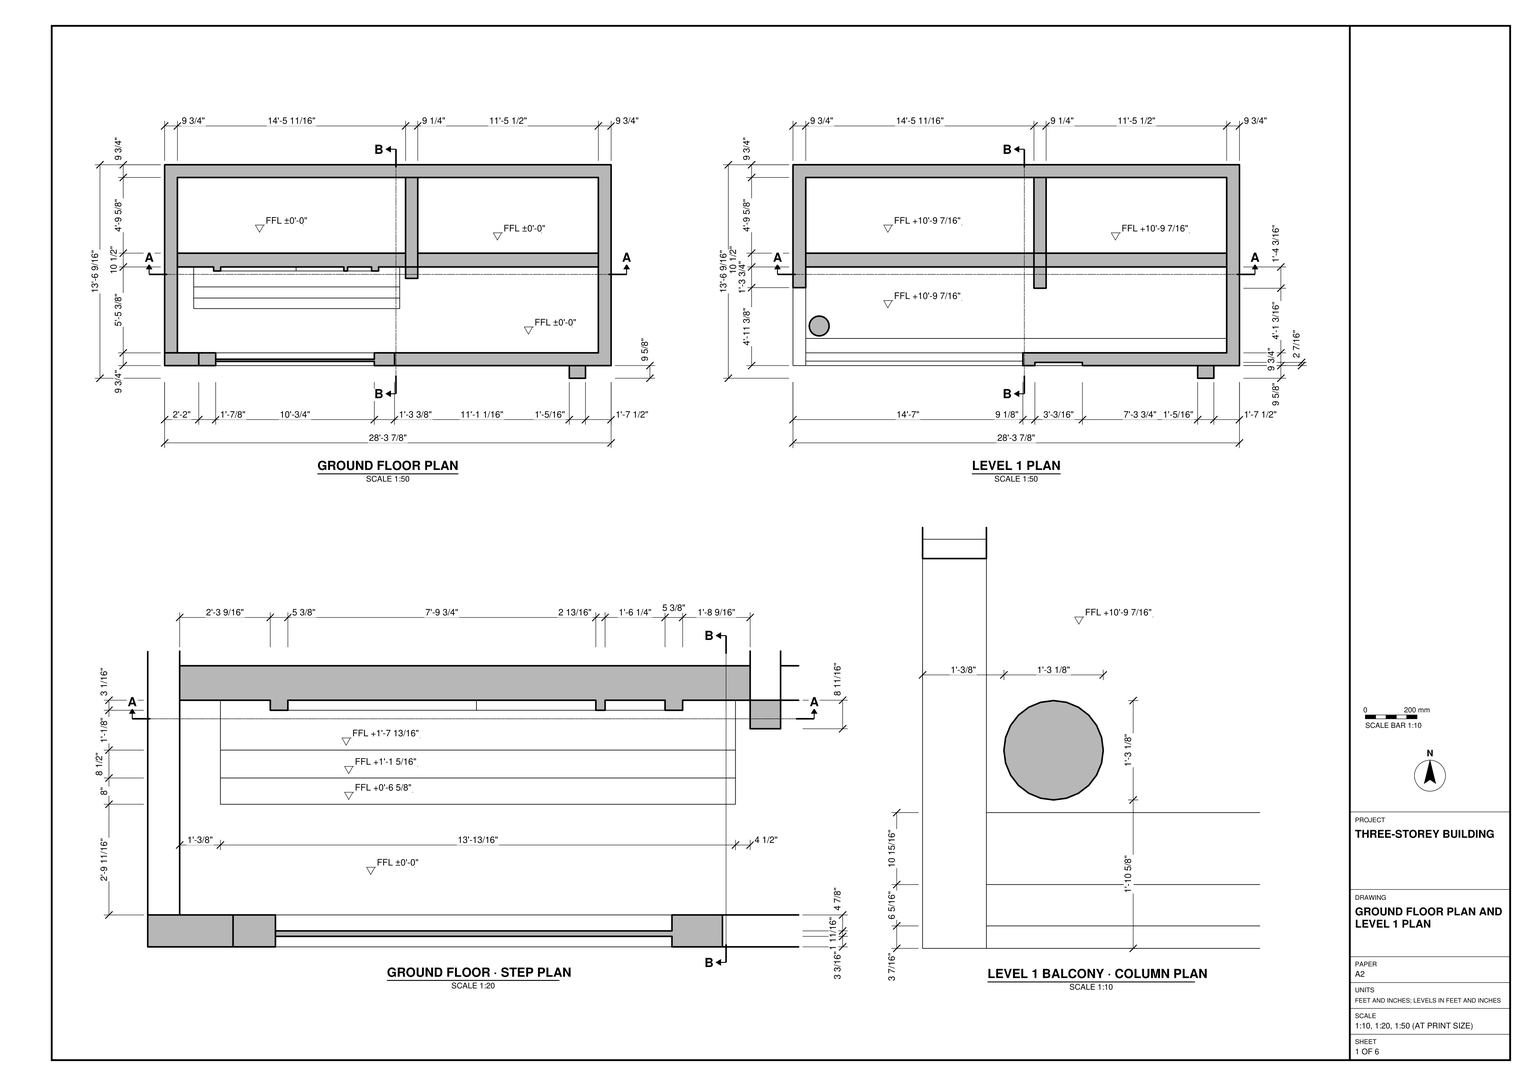
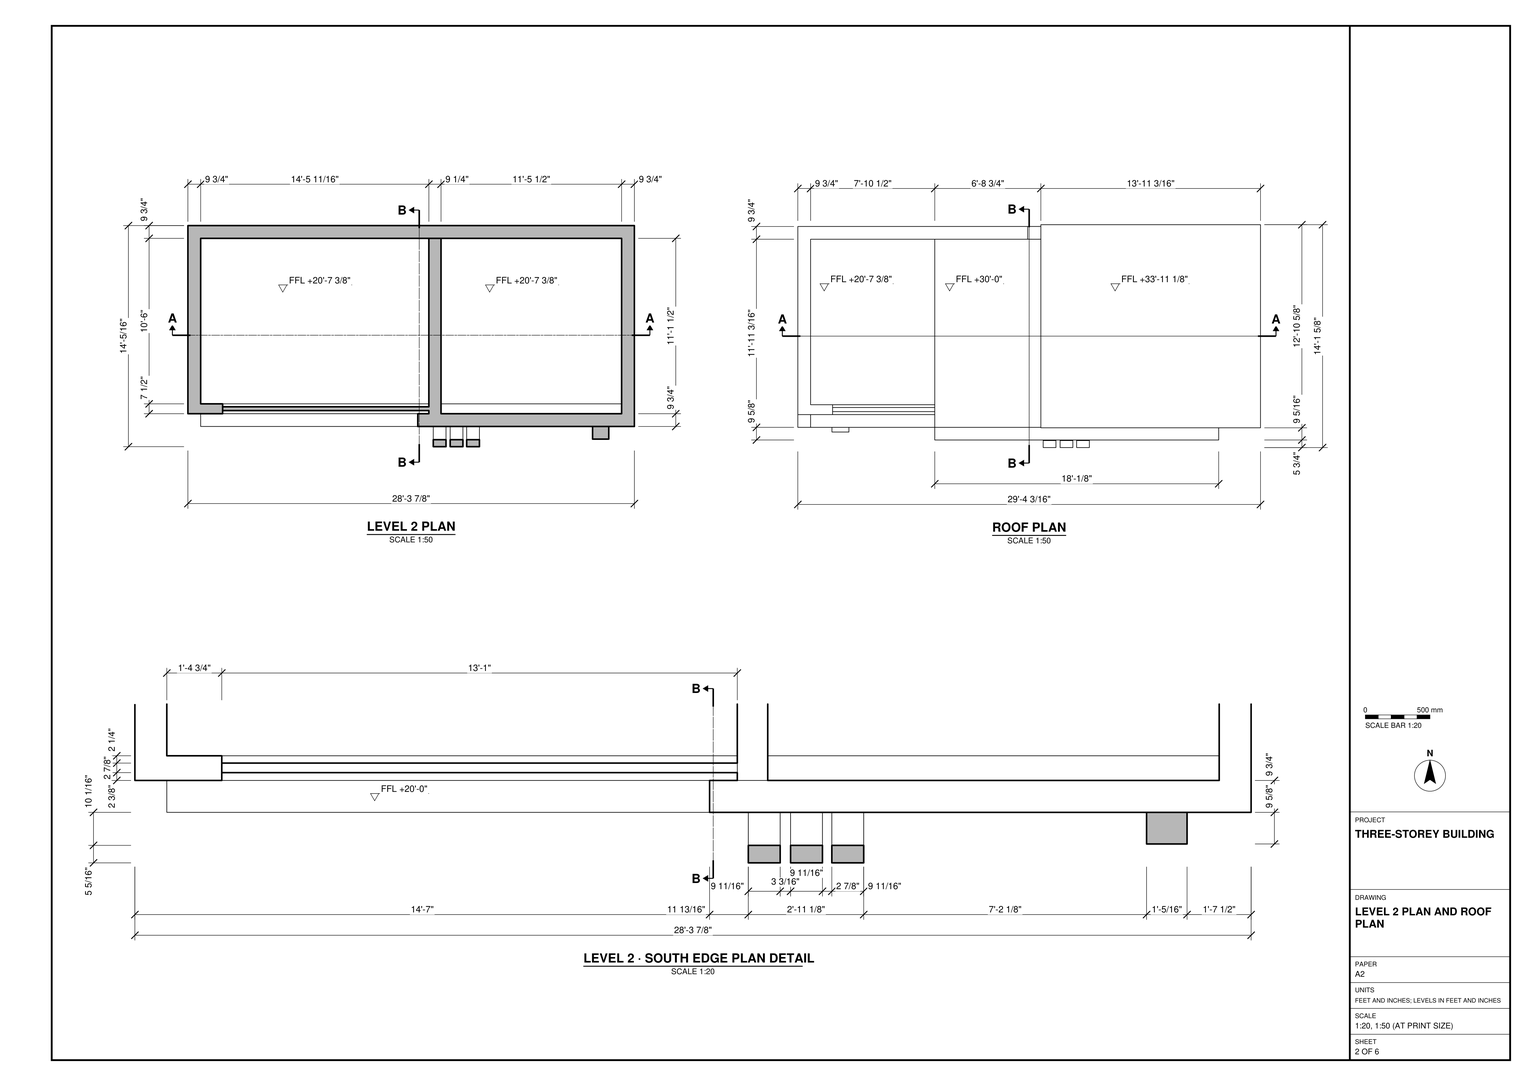
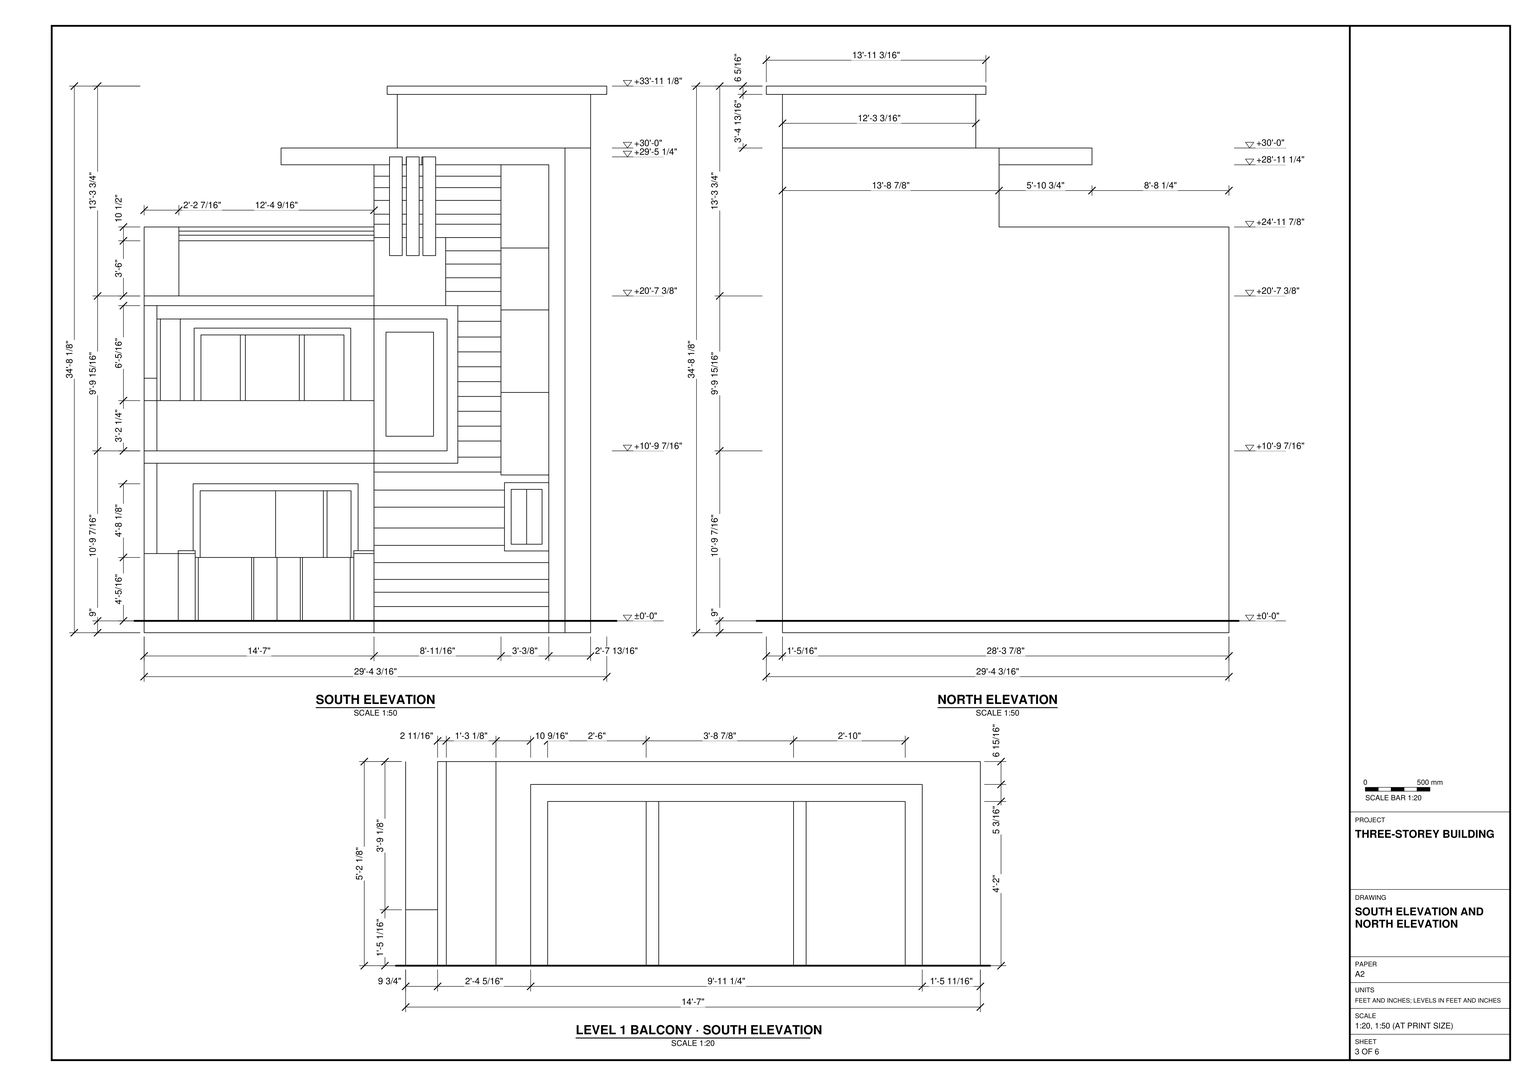
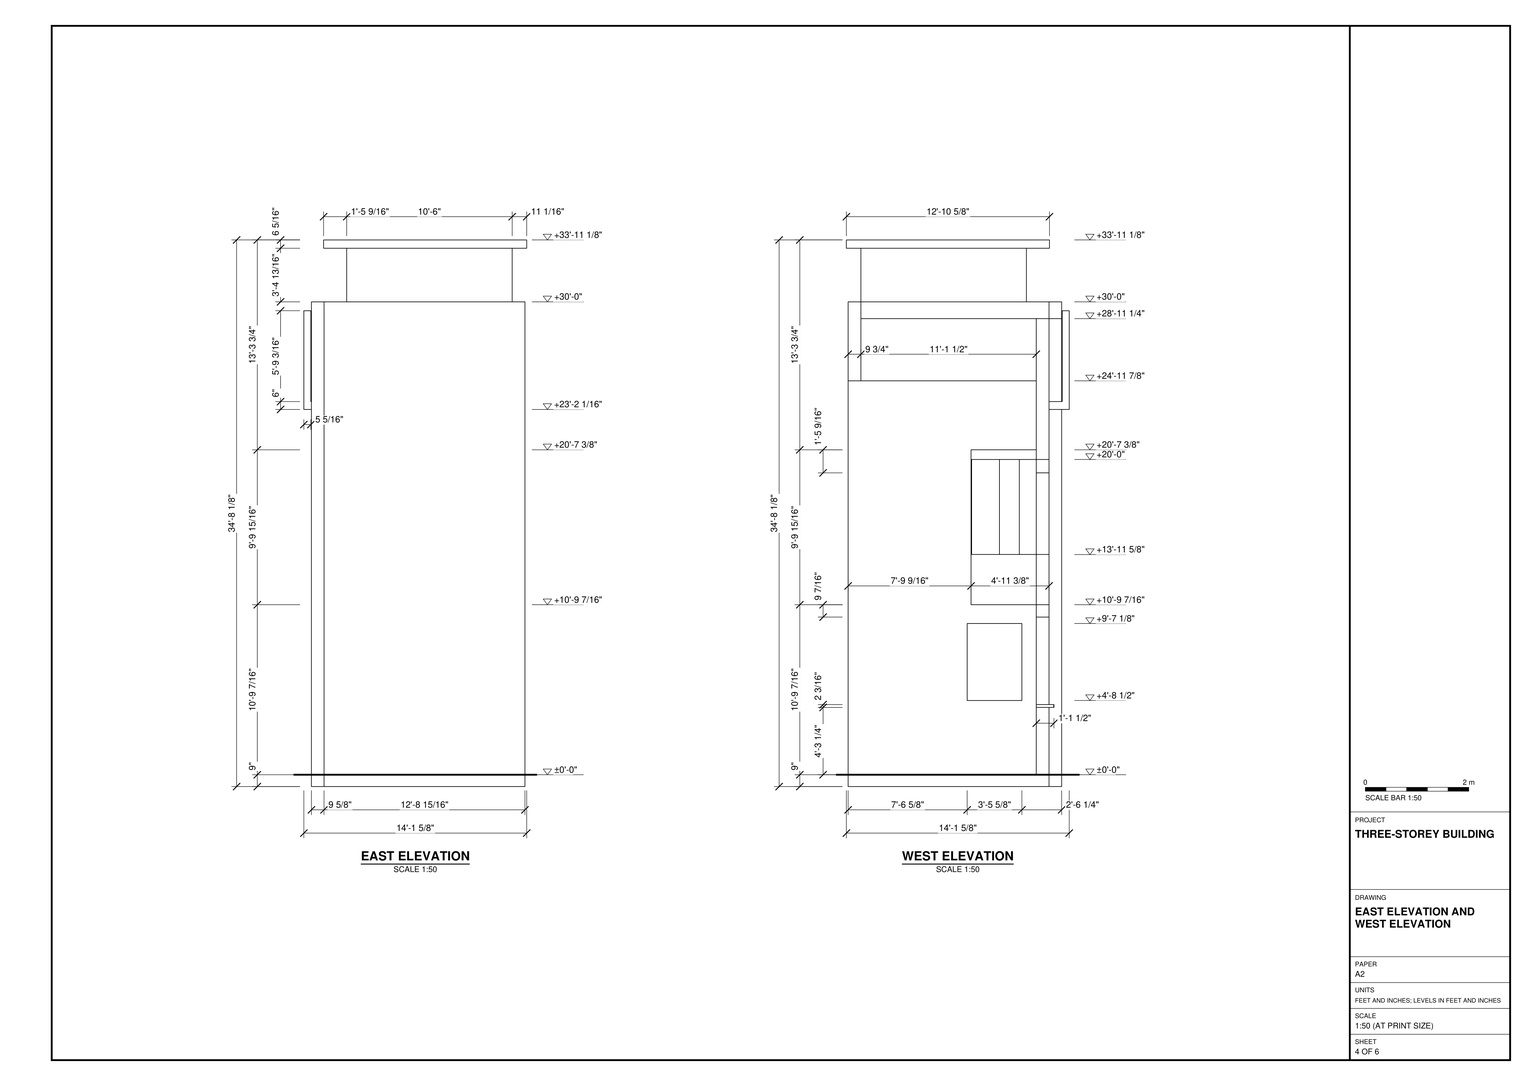
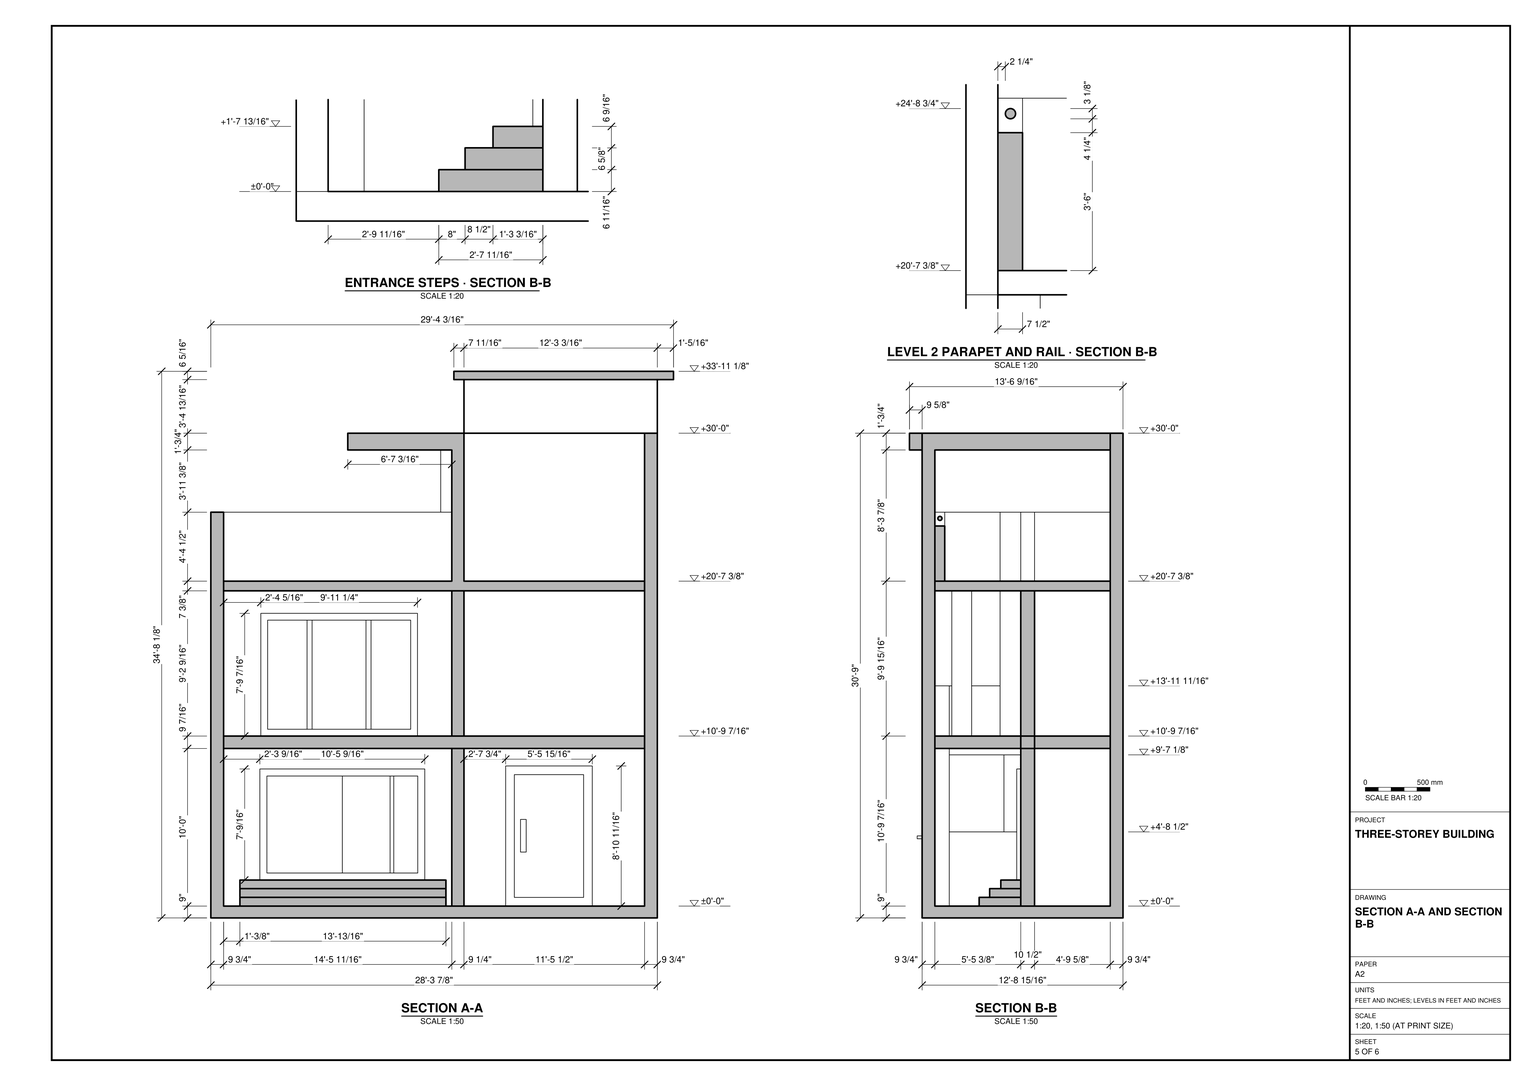
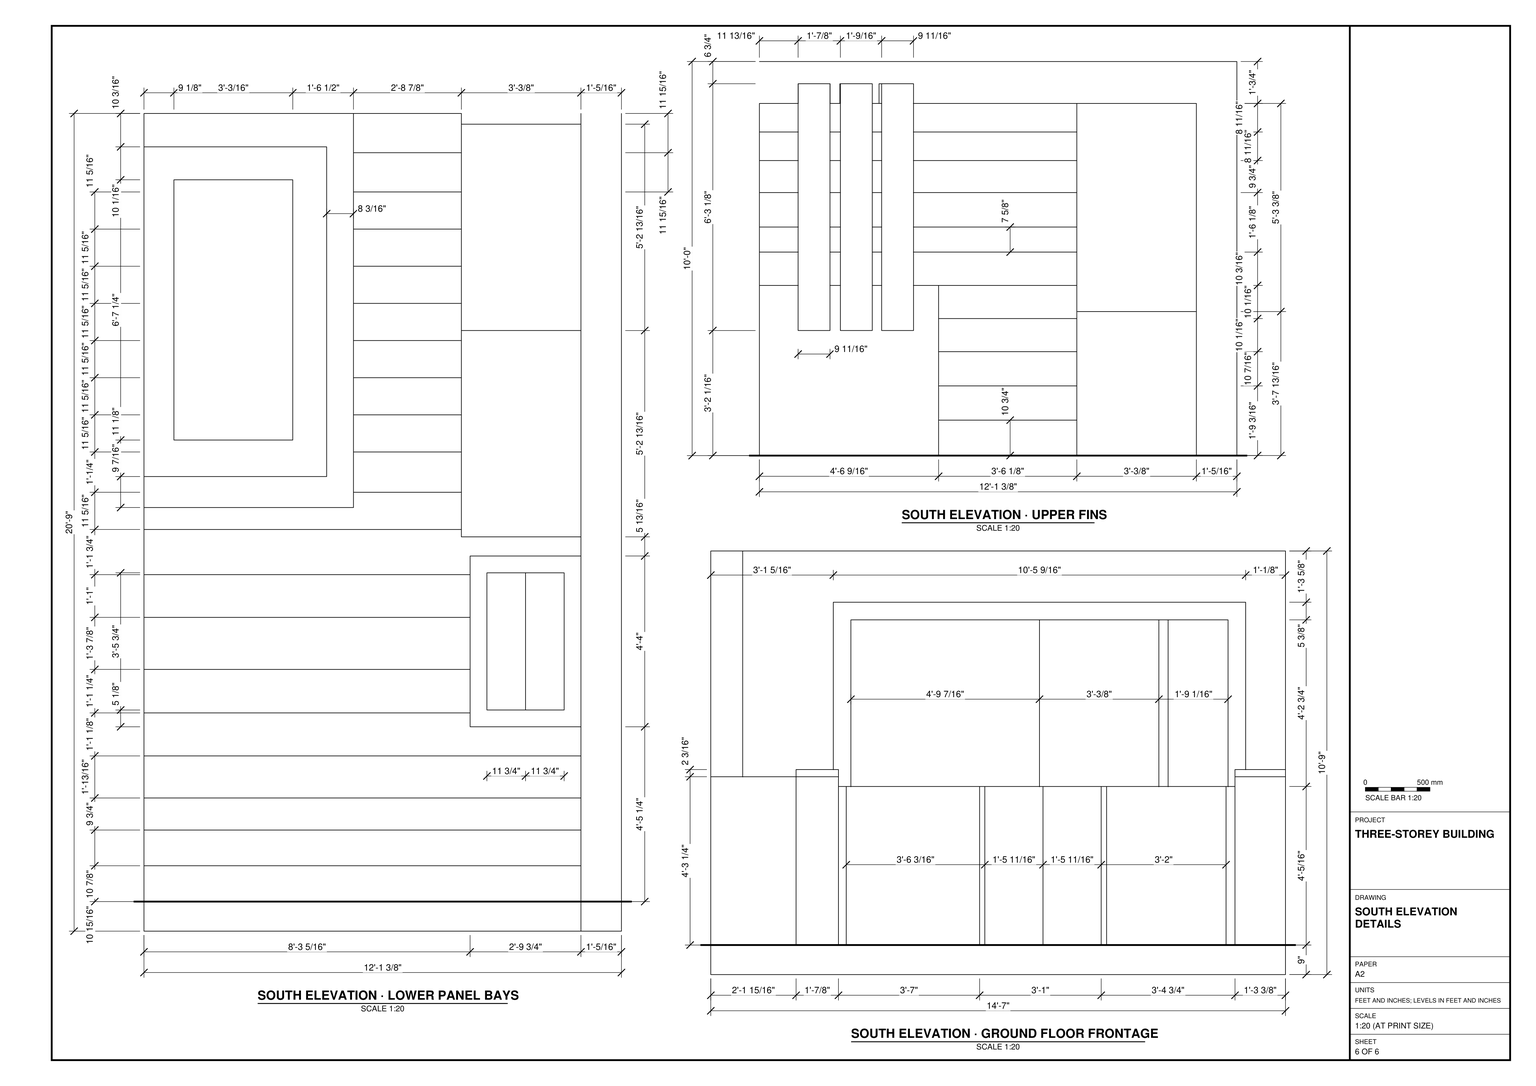
Build the three-storey building in SketchUp using task_files/diagram_01.pdf. Work in feet and inches. Set the overall dimensions to 29'-4 3/16" along the south elevation, 14'-1 5/8" from south to north and 34'-8 1/8" from the underside of the base to the top of the roof. Set the finished floor levels to ±0'-0", +10'-9 7/16" and +20'-7 3/8".

Lay out the exterior walls, internal divisions and floor slabs from the plans, keeping the wall thicknesses as drawn. In the south-west bay, model the broad ground-floor steps and the recessed balcony above them. Use the enlarged details to place the balcony column, parapet and framed opening. Follow the south elevation for the smaller ground-floor window, the projecting rectangular surround at balcony level, the horizontal bands and the three upper vertical fins. Model the open terrace and the two flat roof slabs at their distinct heights, retaining the overhangs shown in plan and elevation.

Keep walls, floor slabs and roofs in separate groups or components. Keep each furniture or joinery piece shown separate and use components for repeated parts. Any decor or loose items shown may be represented by suitable library components. Save one SketchUp model as output_files/three_storey_building_with_a_balcony_and_stepped_roof.skp.

# SketchUp Ruby script. Lengths in inches.
U = 1.inch
M = Sketchup.active_model
def pt(a) = Geom::Point3d.new(a.map { |v| v * U })
def face(e, loops, mat)
  f = e.add_face(loops[0].map { |a| pt(a) })
  loops[1..].each { |l| e.add_face(l.map { |a| pt(a) }).erase! }
  f.material = f.back_material = mat if mat
  f
end
# faces: each face lists its corners as indices into pts; further lists are holes
def faces(e, pts, list, mat = nil) = list.each { |f| face(e, (f[0].is_a?(Array) ? f : [f]).map { |l| l.map { |i| pts[i] } }, mat) }
# xy, xz, yz: faces in a plane at the given z, y or x. An outline is a flat list of corners, or four numbers for a rectangle; further outlines are holes
def ring(l) = l.size == 4 ? [[l[0], l[1]], [l[2], l[1]], [l[2], l[3]], [l[0], l[3]]] : l.each_slice(2).to_a
def flat(e, list, mat, &to3) = list.each { |f| face(e, (f[0].is_a?(Array) ? f : [f]).map { |l| ring(l).map { |u, v| to3.(u, v) } }, mat) }
def xy(e, z, list, mat = nil) = flat(e, list, mat) { |x, y| [x, y, z] }
def xz(e, y, list, mat = nil) = flat(e, list, mat) { |x, z| [x, y, z] }
def yz(e, x, list, mat = nil) = flat(e, list, mat) { |y, z| [x, y, z] }
def lines(e, pts, list) = list.each { |a, b| e.add_line(pt(pts[a]), pt(pts[b])) }
# prism: a flat outline (further loops are holes) pulled along v
def prism(e, loops, v, mat = nil)
  f = face(e, loops, mat); d = Geom::Vector3d.new(v.map { |x| x * U })
  f.pushpull(f.normal.samedirection?(d) ? d.length : -d.length)
end
def box(e, o, s, mat = nil) = prism(e, [[o, [o[0] + s[0], o[1], o[2]], [o[0] + s[0], o[1] + s[1], o[2]], [o[0], o[1] + s[1], o[2]]]], [0, 0, s[2]], mat)
def at(x, y, z, deg = 0) = Geom::Transformation.translation(pt([x, y, z])) * Geom::Transformation.rotation(ORIGIN, Z_AXIS, deg.degrees)
def axes(o, x, y, z) = Geom::Transformation.new([*x, 0, *y, 0, *z, 0, *pt(o).to_a, 1])
def part(name) = M.definitions.add(name)
# library, detail: a bought-in or finely detailed component or shape, given as its bounding box
def library(name, o, s) = part(name).tap { |d| box(d.entities, o, s) }
def detail(e, o, s) = box(e.add_group.entities, o, s)
def put(e, d, t, mat = nil) = e.add_instance(d, t).tap { |i| i.material = mat if mat }
def group(e, t, mat = nil) = e.add_group.tap { |g| g.transformation = t; g.material = mat if mat }.entities
root = M.entities
M.materials.add("[0012_Bisque]").color = [255, 228, 196]
M.materials.add("[Blinds Cellular White]").color = [217, 211, 213]
M.materials.add("[Blinds Cloth Horizontal]").color = [192, 163, 85]
M.materials.add("[Blinds Vertical Stripe Gray]").color = [160, 160, 160]
M.materials.add("[Blinds Weave]").color = [141, 91, 25]
M.materials.add("[Blinds Wood Light]").color = [155, 100, 14]
M.materials.add("[Carpet Diamond Olive]").color = [87, 77, 61]
M.materials.add("[Carpet Pattern Leaf Squares Tan]").color = [181, 154, 125]
M.materials.add("[Color M07]").color = [58, 58, 58]
M.materials.add("[Color M08]").color = [30, 30, 30]
M.materials.add("[Concrete Tile]").color = [203, 190, 164]
M.materials.add("[Formica Beige]").color = [211, 187, 149]
M.materials.add("[Formica Graystone]").color = [149, 146, 135]
M.materials.add("[Formica Laminate Dark]").color = [50, 53, 60]
M.materials.add("[Formica Laminate Light]").color = [213, 189, 164]
M.materials.add("[Formica Speckled Grey]").color = [94, 105, 111]
M.materials.add("[Metal Embossed]").color = [144, 144, 144]
M.materials.add("[Quartz Light Brown]").color = [199, 184, 152]
M.materials.add("[Stone Marble]").color = [143, 138, 136]
M.materials.add("[Translucent Glass Blue]").color = [100, 149, 237]
M.materials["[Translucent Glass Blue]"].alpha = 0.5
M.materials.add("[Translucent Glass Safety]").color = [204, 235, 244]
M.materials["[Translucent Glass Safety]"].alpha = 0.5
M.materials.add("[Wood Bamboo]").color = [177, 105, 43]
M.materials.add("[Wood Cherry Original]").color = [152, 86, 42]
M.materials.add("[Wood Floor Light]").color = [204, 176, 127]
M.materials.add("[Wood Floor Parquet]").color = [145, 89, 39]
xy(root,0,[[308.06,5.75,320.39,15.375],[0,15.375,339.89,168.31]])
xy(root,9,[[0,15.375,25.97,25.09],[25.97,15.375,38.88,25.09],[159.625,15.375,175,25.09],[38.88,18.58,159.625,20.23],[38.88,20.23,159.625,25.09],
  [22.12,58.79,178.96,90.48],[183.43,81.79,192.7,90.48],[9.72,90.48,183.43,100.97],[183.43,90.48,192.7,158.59],[192.7,90.48,330.17,100.97],
  [9.72,100.97,183.43,158.59],[192.7,100.97,330.17,158.59]])
xy(root,9,[[38.88,15.375,159.625,18.58]],"[0012_Bisque]")
xy(root,9,[[9.72,25.09,330.17,25.09,330.17,90.48,192.7,90.48,192.7,81.79,183.43,81.79,183.43,90.48,178.96,90.48,178.96,58.79,22.12,58.79,22.12,90.48,9.72,90.48]],"[Carpet Pattern Leaf Squares Tan]")
xy(root,15.65,[[22.12,66.79,178.96,90.48]])
xy(root,15.65,[[22.12,58.79,178.96,66.79]],"[Concrete Tile]")
xy(root,22.3,[[22.12,75.29,178.96,90.48]])
xy(root,22.3,[[22.12,66.79,178.96,75.29]],"[Concrete Tile]")
xy(root,28.83,[[37.31,87.42,162.87,90.48]])
xy(root,28.83,[[22.12,75.29,178.96,75.29,178.96,90.48,162.87,90.48,162.87,87.42,37.31,87.42,37.31,90.48,22.12,90.48]],"[Concrete Tile]")
xy(root,34.18,[[42.67,87.42,100.09,90.48],[100.09,87.42,136.45,90.48],[139.26,87.42,157.52,90.48]],"[Formica Laminate Dark]")
xy(root,57.28,[[38.88,18.58,159.625,20.23]],"[Color M08]")
xy(root,60.25,[[159.625,11.625,175,15.375],[25.97,11.8125,38.88,15.375],[159.625,15.375,175,25.09]])
xy(root,60.25,[[0,15.375,25.97,25.09]],"[0012_Bisque]")
xy(root,62.4375,[[159.625,11.625,175,25.09],[25.97,11.8125,38.88,25.09]],"[0012_Bisque]")
xy(root,65.5,[[0,36.05,9.72,77.67]],"[0012_Bisque]")
xy(root,108.03,[[42.67,87.42,100.09,90.48],[100.09,87.42,136.45,90.48],[139.26,87.42,157.52,90.48]],"[Formica Laminate Dark]")
xy(root,113.39,[[37.31,87.42,162.87,90.48]])
xy(root,124.14,[[0,36.05,9.72,77.67]])
xy(root,129,[[183.43,81.79,192.7,90.48],[192.7,81.79,330.17,90.48],[9.72,90.48,183.43,100.97],[183.43,90.48,192.7,100.97],[192.7,90.48,330.17,100.97],
  [9.72,100.97,183.43,158.59],[183.43,100.97,192.7,158.59],[192.7,100.97,330.17,158.59]])
xy(root,129,[[0,15.375,0,25.09,9.72,25.09,9.72,90.48,183.43,90.48,183.43,81.79,330.17,81.79,330.17,25.09,175,25.09,175,15.375]],"[Formica Laminate Light]")
xy(root,138.4375,[[0,15.375,9.72,74.73],[9.72,18.8,175,25.09],[9.72,25.09,330.17,36.05],[19.94,37.98,17.99,38.24,16.16,38.99,14.6,40.2,13.4,41.76,12.64,43.59,12.38,45.54,12.64,47.5,13.4,49.32,14.6,50.89,16.16,52.09,17.99,52.85,19.94,53.11,21.9,52.85,23.73,52.09,25.29,50.89,26.49,49.32,27.25,47.5,27.51,45.54,27.25,43.59,26.49,41.76,25.29,40.2,23.73,38.99,21.9,38.24],[183.43,74.29,192.7,90.48],
  [9.72,90.48,183.43,100.97],[183.43,90.48,192.7,100.97],[192.7,90.48,330.17,100.97],[9.72,100.97,183.43,158.59],[183.43,100.97,192.7,158.59],
  [192.7,100.97,330.17,158.59]])
xy(root,138.4375,[[9.72,15.375,175,18.8]],"[0012_Bisque]")
xy(root,138.4375,[[[9.72,36.05,330.17,36.05,330.17,90.48,192.7,90.48,192.7,74.29,183.43,74.29,183.43,90.48,9.72,90.48],[19.94,37.98,17.99,38.24,16.16,38.99,14.6,40.2,13.4,41.76,12.64,43.59,12.38,45.54,12.64,47.5,13.4,49.32,14.6,50.89,16.16,52.09,17.99,52.85,19.94,53.11,21.9,52.85,23.73,52.09,25.29,50.89,26.49,49.32,27.25,47.5,27.51,45.54,27.25,43.59,26.49,41.76,25.29,40.2,23.73,38.99,21.9,38.24]]],"[Carpet Diamond Olive]")
xy(root,149.55,[[184.12,15.375,220.3,17.8125]])
xy(root,176.6875,[[0,15.375,9.72,74.73],[9.72,18.8,175,25.09]],"[Translucent Glass Safety]")
xy(root,228.8,[[184.12,15.375,220.3,17.8125]])
xy(root,238.84,[[9.72,15.375,175,25.09]],"[Formica Laminate Light]")
xy(root,249,[[183.43,25.09,192.7,74.29],[192.7,25.09,330.17,90.48],[19.94,37.98,21.9,38.24,23.73,38.99,25.29,40.2,26.49,41.76,27.25,43.59,27.51,45.54,27.25,47.5,26.49,49.32,25.29,50.89,23.73,52.09,21.9,52.85,19.94,53.11,17.99,52.85,16.16,52.09,14.6,50.89,13.4,49.32,12.64,47.5,12.38,45.54,12.64,43.59,13.4,41.76,14.6,40.2,16.16,38.99,17.99,38.24],[183.43,74.29,192.7,90.48],[9.72,90.48,183.43,100.97],
  [183.43,90.48,192.7,100.97],[192.7,90.48,330.17,100.97],[9.72,100.97,183.43,158.59],[183.43,100.97,192.7,158.59],[192.7,100.97,330.17,158.59]])
xy(root,249,[[9.72,15.375,175,25.09]],"[0012_Bisque]")
xy(root,249,[[0,25.09,0,74.73,9.72,74.73,9.72,90.48,183.43,90.48,183.43,25.09]],"[Formica Laminate Light]")
xy(root,256.375,[[0,25.09,0,74.73,9.72,74.73,9.72,32.61,26.45,32.61,26.45,25.09],[26.45,25.09,183.43,32.61],[192.7,25.09,330.17,32.61],[9.72,32.61,183.43,158.59],[192.7,32.61,330.17,158.59]])
xy(root,287.09,[[186.78,0,196.49,15.375],[199.66,0,209.37,15.375],[212.22,0,221.93,15.375]])
xy(root,293.09,[[186.78,5.33,196.49,15.375],[199.66,5.33,209.37,15.375],[212.22,5.33,221.93,15.375]],"[Formica Speckled Grey]")
xy(root,298.375,[[26.45,25.09,183.43,32.61]],"[Translucent Glass Safety]")
xy(root,308.875,[[0,25.09,26.45,25.09,26.45,32.61,9.72,32.61,9.72,158.59,175,158.59,175,168.31,0,168.31]],"[0012_Bisque]")
xy(root,356.24,[[104.25,5.75,308.06,15.375],[104.25,15.375,175,25.09],[104.25,25.09,183.43,158.59]],"[Formica Laminate Light]")
xy(root,362.24,[[186.78,0,196.49,5.33],[199.66,0,209.37,5.33],[212.22,0,221.93,5.33]],"[Formica Speckled Grey]")
xy(root,369,[[104.25,5.75,320.39,15.375],[192.7,32.61,330.17,158.59],[330.17,32.61,339.89,158.59]])
xy(root,369,[[175,158.59,339.89,168.31]],"[Formica Beige]")
xy(root,369,[[104.25,15.375,339.89,15.375,339.89,25.09,192.7,25.09,192.7,158.59,104.25,158.59],[192.7,25.09,330.17,32.61],[330.17,25.09,339.89,32.61]],"[Formica Graystone]")
xy(root,409.8125,[[185.01,15.04,352.2,32.61],[185.01,32.61,192.7,169.65],[192.7,32.61,339.89,158.59],[339.89,32.61,352.2,169.65],[192.7,158.59,339.89,169.65]])
xy(root,416.125,[[185.01,15.04,352.2,169.65]],"[Quartz Light Brown]")
xz(root,0,[[186.78,287.09,196.49,362.24],[199.66,287.09,209.37,362.24],[212.22,287.09,221.93,362.24]],"[Formica Speckled Grey]")
xz(root,5.33,[[186.78,293.09,196.49,362.24],[199.66,293.09,209.37,362.24],[212.22,293.09,221.93,362.24]])
xz(root,5.75,[[308.06,0,320.39,0,320.39,369,104.25,369,104.25,356.24,186.82,356.24,186.82,362.24,196.52,362.24,196.52,356.24,199.5,356.24,199.5,362.24,209.21,362.24,209.21,356.24,211.43,356.24,211.43,362.24,221.13,362.24,221.13,356.24,308.06,356.24],[186.82,356.24,196.52,362.24],[199.5,356.24,209.21,362.24],[211.43,356.24,221.13,362.24]])
xz(root,11.625,[[159.625,60.25,175,62.4375]],"[0012_Bisque]")
xz(root,11.8125,[[25.97,60.25,38.88,62.4375]],"[0012_Bisque]")
xz(root,15.04,[[185.01,409.8125,352.2,416.125]],"[Quartz Light Brown]")
xz(root,15.375,[[308.06,0,308.06,356.24,104.25,356.24,104.25,369,320.39,369,320.39,0],[[274.31,62.23,308.06,114.23],[279.42,67.35,302.95,109.12]],[[175,138.4375,230.625,238.84],[184.12,149.55,220.3,228.8]],[186.78,287.09,196.49,293.09],[199.66,287.09,209.37,293.09],
  [212.22,287.09,221.93,293.09]])
xz(root,15.375,[[0,9,25.97,60.25],[25.97,9,38.88,60.25],[159.625,9,175,60.25],[0,129,175,138.4375],[175,129,238.79,129,238.79,249,175,249,175,238.84,230.625,238.84,230.625,138.4375,175,138.4375],
  [9.72,238.84,175,249]],"[0012_Bisque]")
xz(root,15.375,[[279.42,67.35,291.18,109.12],[291.18,67.35,302.95,109.12]],"[Blinds Vertical Stripe Gray]")
xz(root,15.375,[[320.39,0,339.89,369],[[175,249,229.56,300.8125],[186.78,287.09,196.49,293.09],[199.66,287.09,209.37,293.09],[212.22,287.09,221.93,293.09]]],"[Formica Graystone]")
xz(root,15.375,[[271.65,120.07,308.06,182.9],[271.65,182.9,308.06,245.73],[271.65,245.73,308.06,292.86],[271.65,292.86,308.06,356.24]],"[Translucent Glass Blue]")
xz(root,15.375,[[0,138.4375,9.72,176.6875]],"[Translucent Glass Safety]")
xz(root,15.375,[[0,0,175,9],[175,0,308.06,9],[175,9,308.06,19.92],[175,19.92,308.06,30.79],[175,30.79,308.06,40.55],
  [175,40.55,308.06,53.37],[175,53.37,308.06,53.37,308.06,62.23,274.31,62.23,274.31,66.46,175,66.46],[175,66.46,274.31,79.71],[175,79.71,274.31,95.55],[175,95.55,274.31,108.5625],
  [175,108.5625,274.31,108.5625,274.31,114.23,308.06,114.23,308.06,120.07,271.65,120.07,271.65,122.3125,175,122.3125],[175,122.3125,271.65,122.3125,271.65,133.65,238.79,133.65,238.79,129,175,129],[238.79,133.65,271.65,145.92],[238.79,145.92,271.65,157.23],[238.79,157.23,271.65,168.54],
  [238.79,168.54,271.65,179.85],[238.79,179.85,271.65,191.17],[238.79,191.17,271.65,202.48],[238.79,202.48,271.65,213.79],[238.79,213.79,271.65,225.1],
  [238.79,225.1,271.65,237.05],[238.79,237.05,271.65,249],[229.56,249,271.65,259.8],[229.56,259.8,271.65,270.23],[229.56,270.23,271.65,280.64],
  [229.56,280.64,271.65,290.73],[229.56,290.73,271.65,300.8125],[175,300.8125,271.65,310.97],[175,310.97,271.65,318.6],[175,318.6,271.65,329.1],
  [175,329.1,271.65,338.85],[175,338.85,271.65,347.54],[175,347.54,271.65,356.24]],"[Wood Bamboo]")
xz(root,17.8125,[[184.12,149.55,220.3,228.8]],"[Stone Marble]")
xz(root,18.58,[[41.25,9,81.86,57.28],[120.53,9,156.9,57.28]],"[Blinds Wood Light]")
xz(root,18.58,[[38.88,9,41.25,57.28],[81.86,9,83.45,57.28],[118.88,9,120.53,57.28],[156.9,9,159.625,57.28]],"[Color M07]")
xz(root,18.58,[[83.45,9,101.16,57.28],[101.16,9,118.88,57.28]],"[Metal Embossed]")
xz(root,18.8,[[9.72,138.4375,175,176.6875]],"[Translucent Glass Safety]")
xz(root,20.23,[[38.88,9,159.625,57.28]],"[0012_Bisque]")
xz(root,25.09,[[0,9,9.72,60.25],[159.625,9,175,60.25],[175,9,330.17,129],[159.625,60.25,175,62.4375],[175,129,330.17,138.4375],
  [175,138.4375,175,238.84,9.72,238.84,9.72,249,330.17,249,330.17,138.4375],[175,249,183.43,256.375],[183.43,249,192.7,256.375],[192.7,249,330.17,256.375],[175,256.375,183.43,298.375],
  [192.7,256.375,330.17,369],[175,298.375,183.43,356.24]])
xz(root,25.09,[[9.72,9,25.97,60.25],[25.97,9,38.88,62.4375],[0,60.25,9.72,129],[0,249,175,256.375],[0,256.375,26.45,308.875]],"[0012_Bisque]")
xz(root,25.09,[[9.72,138.4375,175,176.6875],[26.45,256.375,175,298.375]],"[Translucent Glass Safety]")
xz(root,32.61,[[192.7,369,339.89,409.8125]],"[Formica Graystone]")
xz(root,32.61,[[9.72,256.375,26.45,308.875]],"[Quartz Light Brown]")
xz(root,32.61,[[26.45,256.375,183.43,298.375]],"[Translucent Glass Safety]")
xz(root,36.05,[[0,65.5,9.72,124.14]],"[0012_Bisque]")
xz(root,58.79,[[22.12,9,178.96,15.65]],"[Concrete Tile]")
xz(root,66.79,[[22.12,15.65,178.96,22.3]],"[Concrete Tile]")
xz(root,74.29,[[183.43,138.4375,192.7,249]],"[0012_Bisque]")
xz(root,74.73,[[0,138.4375,9.72,176.6875],[0,249,9.72,256.375]])
xz(root,74.73,[[0,176.6875,9.72,193.72],[0,193.72,9.72,249]],"[0012_Bisque]")
xz(root,75.29,[[22.12,22.3,178.96,28.83]],"[Concrete Tile]")
xz(root,77.67,[[0,65.5,9.72,124.14]],"[0012_Bisque]")
xz(root,81.79,[[183.43,9,192.7,129]],"[0012_Bisque]")
xz(root,87.42,[[[37.31,28.83,162.87,113.39],[42.67,34.18,157.52,108.03]],[136.45,34.18,139.26,108.03]],"[Formica Laminate Dark]")
xz(root,90.48,[[22.12,9,178.96,15.65],[183.43,9,192.7,129],[22.12,15.65,178.96,22.3],[22.12,22.3,178.96,28.83],[9.72,129,330.17,138.4375],
  [183.43,138.4375,192.7,249]])
xz(root,90.48,[[121.94,143.62,152.125,226.69]],"[Blinds Cellular White]")
xz(root,90.48,[[43.24,143.62,73.24,226.69]],"[Blinds Cloth Horizontal]")
xz(root,90.48,[[77.07,143.62,118.12,226.69]],"[Blinds Weave]")
xz(root,90.48,[[[38.06,138.4375,157.31,231.875],[43.24,143.62,152.125,226.69]],[73.24,143.62,77.07,226.69],[118.12,143.62,121.94,226.69]],"[Formica Laminate Dark]")
xz(root,90.48,[[9.72,9,22.12,9,22.12,28.83,37.31,28.83,37.31,113.39,162.87,113.39,162.87,28.83,178.96,28.83,178.96,9,183.43,9,183.43,129,9.72,129],[192.7,9,224.4375,9,224.4375,115.6875,290.375,115.6875,290.375,9,330.17,9,330.17,129,192.7,129],[9.72,138.4375,38.06,138.4375,38.06,231.875,157.31,231.875,157.31,138.4375,183.43,138.4375,183.43,249,9.72,249],[192.7,138.4375,330.17,249]],"[Formica Laminate Light]")
xz(root,90.48,[[[224.4375,9,290.375,115.6875],[231.04,15.61,283.77,109.08]]],"[Formica Speckled Grey]")
xz(root,90.48,[[[231.04,15.61,283.77,109.08],[235.75,50.12,240.0625,74.99]]],"[Wood Cherry Original]")
xz(root,90.48,[[235.75,50.12,240.0625,74.99]],"[Wood Floor Light]")
xz(root,90.48,[[42.67,34.18,100.09,108.03],[100.09,34.18,136.45,108.03],[139.26,34.18,157.52,108.03]],"[Wood Floor Parquet]")
xz(root,100.97,[[9.72,9,183.43,129],[192.7,9,330.17,129],[9.72,129,330.17,138.4375],[9.72,138.4375,183.43,249],[183.43,138.4375,192.7,249],
  [192.7,138.4375,330.17,249]])
xz(root,158.59,[[9.72,9,183.43,129],[183.43,9,192.7,129],[192.7,9,330.17,129],[9.72,129,183.43,138.4375],[183.43,129,192.7,138.4375],
  [192.7,129,330.17,138.4375],[9.72,138.4375,183.43,249],[183.43,138.4375,192.7,249],[192.7,138.4375,330.17,249],[9.72,249,183.43,256.375],
  [183.43,249,183.43,356.24,175,356.24,175,369,192.7,369,192.7,249],[192.7,249,330.17,256.375],[192.7,256.375,330.17,369]])
xz(root,158.59,[[9.72,256.375,183.43,308.875],[175,308.875,183.43,356.24]],"[0012_Bisque]")
xz(root,158.59,[[192.7,369,339.89,409.8125]],"[Formica Graystone]")
xz(root,158.59,[[104.25,356.24,175,369]],"[Quartz Light Brown]")
xz(root,168.31,[[0,0,0,308.875,175,308.875,175,369,339.89,369,339.89,0]],"[0012_Bisque]")
xz(root,169.65,[[185.01,409.8125,352.2,416.125]],"[Quartz Light Brown]")
yz(root,0,[[15.375,129,25.09,138.4375]])
yz(root,0,[[[15.375,0,15.375,9,25.09,9,25.09,138.4375,74.73,138.4375,74.73,256.375,25.09,256.375,25.09,308.875,168.31,308.875,168.31,0],[36.05,65.5,77.67,124.14]],[15.375,9,25.09,60.25],[25.09,249,74.73,256.375]],"[0012_Bisque]")
yz(root,0,[[15.375,138.4375,25.09,176.6875],[25.09,138.4375,74.73,176.6875]],"[Translucent Glass Safety]")
yz(root,9.72,[[25.09,9,36.05,129],[90.48,9,100.97,129],[100.97,9,158.59,129],[36.05,124.14,90.48,129],[36.05,129,74.73,138.4375],
  [74.73,129,90.48,138.4375],[90.48,129,100.97,138.4375],[100.97,129,158.59,138.4375],[18.8,138.4375,25.09,176.6875],[74.73,138.4375,90.48,249],
  [90.48,138.4375,100.97,249],[100.97,138.4375,158.59,249],[74.73,249,90.48,256.375],[90.48,249,100.97,256.375],[100.97,249,158.59,256.375]])
yz(root,9.72,[[15.375,238.84,25.09,249],[32.61,256.375,74.73,308.875],[74.73,256.375,90.48,308.875],[90.48,256.375,100.97,308.875],[100.97,256.375,158.59,308.875]],"[0012_Bisque]")
yz(root,9.72,[[36.05,9,90.48,65.5],[77.67,65.5,90.48,124.14]],"[Formica Laminate Light]")
yz(root,9.72,[[15.375,138.4375,18.8,176.6875],[25.09,138.4375,36.05,176.6875],[36.05,138.4375,74.73,176.6875]],"[Translucent Glass Safety]")
yz(root,22.12,[[58.79,9,90.48,15.65],[66.79,15.65,90.48,22.3],[75.29,22.3,90.48,28.83]],"[Concrete Tile]")
yz(root,25.97,[[15.375,9,25.09,60.25]])
yz(root,25.97,[[11.8125,60.25,25.09,62.4375]],"[0012_Bisque]")
yz(root,26.45,[[25.09,256.375,32.61,298.375],[28.93,302.6,28.52,302.65,28.15,302.81,27.82,303.06,27.57,303.38,27.42,303.76,27.37,304.16,27.42,304.57,27.57,304.94,27.82,305.27,28.15,305.52,28.52,305.67,28.93,305.73,29.33,305.67,29.71,305.52,30.03,305.27,30.28,304.94,30.4375,304.57,30.49,304.16,30.4375,303.76,30.28,303.38,30.03,303.06,29.71,302.81,29.33,302.65]])
yz(root,26.45,[[[25.09,298.375,32.61,308.875],[28.93,302.6,28.52,302.65,28.15,302.81,27.82,303.06,27.57,303.38,27.42,303.76,27.37,304.16,27.42,304.57,27.57,304.94,27.82,305.27,28.15,305.52,28.52,305.67,28.93,305.73,29.33,305.67,29.71,305.52,30.03,305.27,30.28,304.94,30.4375,304.57,30.49,304.16,30.4375,303.76,30.28,303.38,30.03,303.06,29.71,302.81,29.33,302.65]]],"[Formica Beige]")
yz(root,37.31,[[87.42,28.83,90.48,113.39]],"[Formica Laminate Dark]")
yz(root,38.88,[[18.58,9,20.23,57.28]])
yz(root,38.88,[[15.375,9,18.58,9,18.58,57.28,20.23,57.28,20.23,9,25.09,9,25.09,60.25,15.375,60.25],[11.8125,60.25,25.09,62.4375]],"[0012_Bisque]")
yz(root,42.67,[[87.42,34.18,90.48,108.03]],"[Formica Laminate Dark]")
yz(root,104.25,[[5.75,356.24,15.375,369]])
yz(root,104.25,[[15.375,356.24,158.59,369]],"[Quartz Light Brown]")
yz(root,136.45,[[87.42,34.18,90.48,108.03]],"[Formica Laminate Dark]")
yz(root,139.26,[[87.42,34.18,90.48,108.03]],"[Formica Laminate Dark]")
yz(root,157.52,[[87.42,34.18,90.48,108.03]],"[Formica Laminate Dark]")
yz(root,159.625,[[15.375,9,15.375,60.25,25.09,60.25,25.09,9,20.23,9,20.23,57.28,18.58,57.28,18.58,9],[11.625,60.25,25.09,62.4375]],"[0012_Bisque]")
yz(root,162.87,[[87.42,28.83,90.48,113.39]])
yz(root,175,[[15.375,9,25.09,60.25],[15.375,60.25,25.09,62.4375],[15.375,129,25.09,138.4375],[15.375,138.4375,15.375,238.84,25.09,238.84,25.09,176.6875,18.8,176.6875,18.8,138.4375],[18.8,138.4375,25.09,176.6875]])
yz(root,175,[[11.625,60.25,15.375,62.4375],[15.375,62.4375,25.09,129],[15.375,249,25.09,356.24],[158.59,308.875,168.31,369]],"[0012_Bisque]")
yz(root,178.96,[[58.79,9,90.48,15.65],[66.79,15.65,90.48,22.3],[75.29,22.3,90.48,28.83]],"[Concrete Tile]")
yz(root,183.43,[[90.48,9,100.97,129],[100.97,9,158.59,129],[90.48,138.4375,100.97,249],[100.97,138.4375,158.59,249],[25.09,256.375,32.61,298.375]])
yz(root,183.43,[[81.79,9,90.48,129],[74.29,138.4375,90.48,249]],"[0012_Bisque]")
yz(root,183.43,[[[32.61,256.375,32.61,298.375,25.09,298.375,25.09,356.24,158.59,356.24,158.59,256.375],[28.93,302.6,29.33,302.65,29.71,302.81,30.03,303.06,30.28,303.38,30.4375,303.76,30.49,304.16,30.4375,304.57,30.28,304.94,30.03,305.27,29.71,305.52,29.33,305.67,28.93,305.73,28.52,305.67,28.15,305.52,27.82,305.27,27.57,304.94,27.42,304.57,27.37,304.16,27.42,303.76,27.57,303.38,27.82,303.06,28.15,302.81,28.52,302.65]]],"[Quartz Light Brown]")
yz(root,184.12,[[15.375,149.55,17.8125,228.8]])
yz(root,185.01,[[15.04,409.8125,169.65,416.125]],"[Quartz Light Brown]")
yz(root,186.78,[[0,287.09,0,362.24,5.33,362.24,5.33,293.09,15.375,293.09,15.375,287.09]],"[Formica Speckled Grey]")
yz(root,192.7,[[81.79,9,90.48,129],[90.48,9,100.97,129],[100.97,9,158.59,129],[74.29,138.4375,90.48,249],[90.48,138.4375,100.97,249],
  [100.97,138.4375,158.59,249],[25.09,256.375,158.59,369]])
yz(root,192.7,[[32.61,369,158.59,409.8125]],"[Formica Graystone]")
yz(root,196.49,[[0,287.09,15.375,287.09,15.375,293.09,5.33,293.09,5.33,362.24,0,362.24]],"[Formica Speckled Grey]")
yz(root,199.66,[[0,287.09,0,362.24,5.33,362.24,5.33,293.09,15.375,293.09,15.375,287.09]],"[Formica Speckled Grey]")
yz(root,209.37,[[0,287.09,15.375,287.09,15.375,293.09,5.33,293.09,5.33,362.24,0,362.24]],"[Formica Speckled Grey]")
yz(root,212.22,[[0,287.09,0,362.24,5.33,362.24,5.33,293.09,15.375,293.09,15.375,287.09]],"[Formica Speckled Grey]")
yz(root,220.3,[[15.375,149.55,17.8125,228.8]])
yz(root,221.93,[[0,287.09,15.375,287.09,15.375,293.09,5.33,293.09,5.33,362.24,0,362.24]],"[Formica Speckled Grey]")
yz(root,308.06,[[5.75,0,15.375,356.24]])
yz(root,320.39,[[5.75,0,15.375,369]])
yz(root,330.17,[[90.48,9,100.97,129],[100.97,9,158.59,129],[25.09,129,81.79,138.4375],[81.79,129,90.48,138.4375],[90.48,129,100.97,138.4375],
  [100.97,129,158.59,138.4375],[90.48,138.4375,100.97,249],[100.97,138.4375,158.59,249],[25.09,249,81.79,256.375],[81.79,249,90.48,256.375],
  [90.48,249,100.97,256.375],[100.97,249,158.59,256.375],[25.09,256.375,158.59,369]])
yz(root,330.17,[[25.09,9,90.48,129],[25.09,138.4375,81.79,249],[81.79,138.4375,90.48,249]],"[Formica Laminate Light]")
yz(root,339.89,[[15.375,0,168.31,369],[32.61,369,158.59,409.8125]],"[Formica Graystone]")
yz(root,352.2,[[15.04,409.8125,169.65,416.125]],"[Quartz Light Brown]")
p = [[17.99,38.24,138.4375],[19.94,37.98,138.4375],[19.94,37.98,249],[17.99,38.24,249],[21.9,38.24,138.4375],[21.9,38.24,249],
  [16.16,38.99,138.4375],[16.16,38.99,249],[23.73,38.99,138.4375],[23.73,38.99,249],[14.6,40.2,138.4375],[14.6,40.2,249],
  [25.29,40.2,138.4375],[25.29,40.2,249],[13.4,41.76,138.4375],[13.4,41.76,249],[26.49,41.76,138.4375],[26.49,41.76,249],
  [12.64,43.59,138.4375],[12.64,43.59,249],[27.25,43.59,138.4375],[27.25,43.59,249],[12.38,45.54,138.4375],[12.38,45.54,249],
  [27.51,45.54,138.4375],[27.51,45.54,249],[12.64,47.5,138.4375],[12.64,47.5,249],[27.25,47.5,138.4375],[27.25,47.5,249],
  [13.4,49.32,138.4375],[13.4,49.32,249],[26.49,49.32,138.4375],[26.49,49.32,249],[14.6,50.89,138.4375],[14.6,50.89,249],
  [25.29,50.89,138.4375],[25.29,50.89,249],[16.16,52.09,138.4375],[16.16,52.09,249],[23.73,52.09,138.4375],[23.73,52.09,249],
  [17.99,52.85,138.4375],[17.99,52.85,249],[21.9,52.85,138.4375],[21.9,52.85,249],[19.94,53.11,138.4375],[19.94,53.11,249],
  [26.45,28.52,302.65],[26.45,28.93,302.6],[183.43,28.93,302.6],[183.43,28.52,302.65],[26.45,29.33,302.65],[183.43,29.33,302.65],
  [26.45,28.15,302.81],[183.43,28.15,302.81],[26.45,29.71,302.81],[183.43,29.71,302.81],[26.45,27.82,303.06],[183.43,27.82,303.06],
  [26.45,30.03,303.06],[183.43,30.03,303.06],[26.45,27.57,303.38],[183.43,27.57,303.38],[26.45,30.28,303.38],[183.43,30.28,303.38],
  [26.45,27.42,303.76],[183.43,27.42,303.76],[26.45,30.4375,303.76],[183.43,30.4375,303.76],[26.45,27.37,304.16],[183.43,27.37,304.16],
  [26.45,30.49,304.16],[183.43,30.49,304.16],[26.45,27.42,304.57],[183.43,27.42,304.57],[26.45,30.4375,304.57],[183.43,30.4375,304.57],
  [26.45,27.57,304.94],[183.43,27.57,304.94],[26.45,30.28,304.94],[183.43,30.28,304.94],[26.45,27.82,305.27],[183.43,27.82,305.27],
  [26.45,30.03,305.27],[183.43,30.03,305.27],[26.45,28.15,305.52],[183.43,28.15,305.52],[26.45,29.71,305.52],[183.43,29.71,305.52],
  [26.45,28.52,305.67],[183.43,28.52,305.67],[26.45,29.33,305.67],[183.43,29.33,305.67],[26.45,28.93,305.73],[183.43,28.93,305.73]]
faces(root,p,[[0,1,2,3],[1,4,5,2],[6,0,3,7],[4,8,9,5],[10,6,7,11],[8,12,13,9],[14,10,11,15],[12,16,17,13],
  [18,14,15,19],[16,20,21,17],[22,18,19,23],[20,24,25,21],[26,22,23,27],[24,28,29,25],[30,26,27,31],[28,32,33,29],
  [34,30,31,35],[32,36,37,33],[38,34,35,39],[36,40,41,37],[42,38,39,43],[40,44,45,41],[46,42,43,47],[44,46,47,45]],"[Formica Speckled Grey]")
faces(root,p,[[48,49,50,51],[49,52,53,50],[54,48,51,55],[52,56,57,53],[58,54,55,59],[56,60,61,57],[62,58,59,63],[60,64,65,61],
  [66,62,63,67],[64,68,69,65],[70,66,67,71],[68,72,73,69],[74,70,71,75],[72,76,77,73],[78,74,75,79],[76,80,81,77],
  [82,78,79,83],[80,84,85,81],[86,82,83,87],[84,88,89,85],[90,86,87,91],[88,92,93,89],[94,90,91,95],[92,94,95,93]],"[Formica Laminate Dark]")
